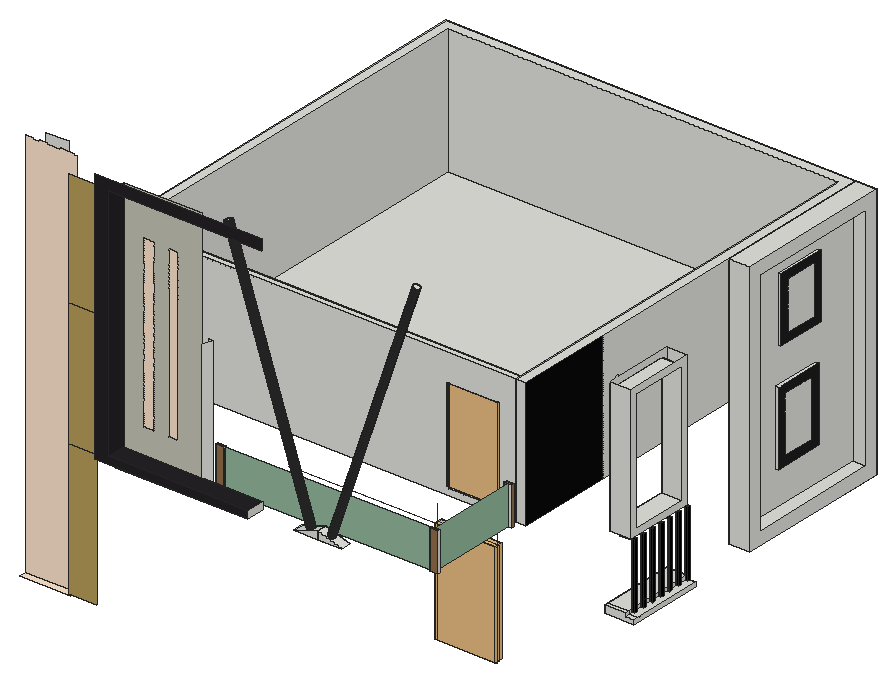
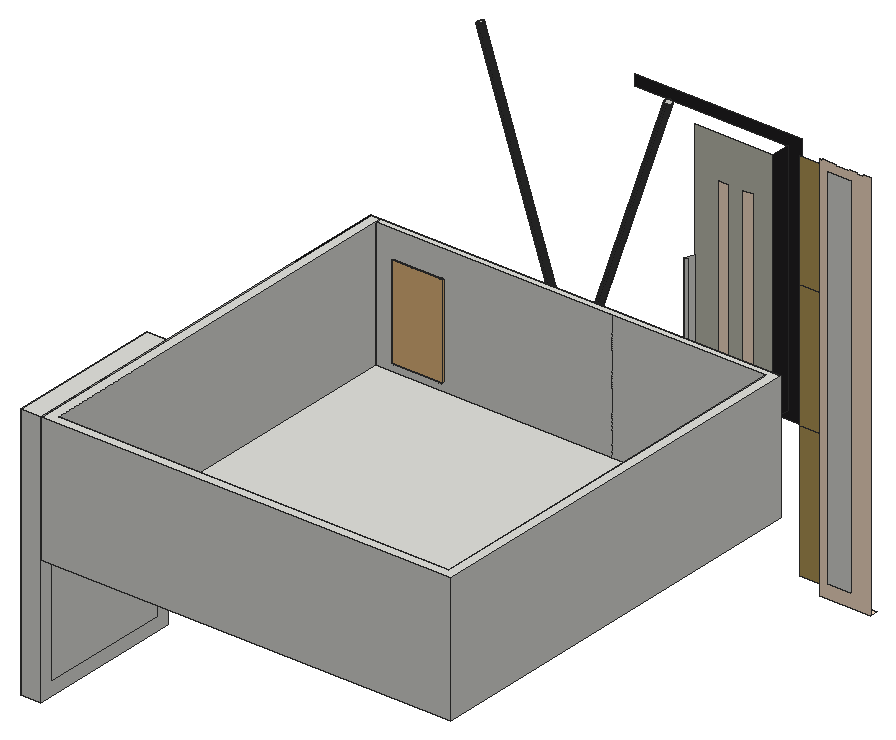
# SketchUp Ruby script. Lengths in inches.
U = 1.inch
M = Sketchup.active_model
def pt(a) = Geom::Point3d.new(a.map { |v| v * U })
def face(e, loops, mat)
  f = e.add_face(loops[0].map { |a| pt(a) })
  loops[1..].each { |l| e.add_face(l.map { |a| pt(a) }).erase! }
  f.material = f.back_material = mat if mat
  f
end
# faces: each face lists its corners as indices into pts; further lists are holes
def faces(e, pts, list, mat = nil) = list.each { |f| face(e, (f[0].is_a?(Array) ? f : [f]).map { |l| l.map { |i| pts[i] } }, mat) }
# xy, xz, yz: faces in a plane at the given z, y or x. An outline is a flat list of corners, or four numbers for a rectangle; further outlines are holes
def ring(l) = l.size == 4 ? [[l[0], l[1]], [l[2], l[1]], [l[2], l[3]], [l[0], l[3]]] : l.each_slice(2).to_a
def flat(e, list, mat, &to3) = list.each { |f| face(e, (f[0].is_a?(Array) ? f : [f]).map { |l| ring(l).map { |u, v| to3.(u, v) } }, mat) }
def xy(e, z, list, mat = nil) = flat(e, list, mat) { |x, y| [x, y, z] }
def xz(e, y, list, mat = nil) = flat(e, list, mat) { |x, z| [x, y, z] }
def yz(e, x, list, mat = nil) = flat(e, list, mat) { |y, z| [x, y, z] }
def lines(e, pts, list) = list.each { |a, b| e.add_line(pt(pts[a]), pt(pts[b])) }
# prism: a flat outline (further loops are holes) pulled along v
def prism(e, loops, v, mat = nil)
  f = face(e, loops, mat); d = Geom::Vector3d.new(v.map { |x| x * U })
  f.pushpull(f.normal.samedirection?(d) ? d.length : -d.length)
end
def box(e, o, s, mat = nil) = prism(e, [[o, [o[0] + s[0], o[1], o[2]], [o[0] + s[0], o[1] + s[1], o[2]], [o[0], o[1] + s[1], o[2]]]], [0, 0, s[2]], mat)
def at(x, y, z, deg = 0) = Geom::Transformation.translation(pt([x, y, z])) * Geom::Transformation.rotation(ORIGIN, Z_AXIS, deg.degrees)
def axes(o, x, y, z) = Geom::Transformation.new([*x, 0, *y, 0, *z, 0, *pt(o).to_a, 1])
def part(name) = M.definitions.add(name)
# library, detail: a bought-in or finely detailed component or shape, given as its bounding box
def library(name, o, s) = part(name).tap { |d| box(d.entities, o, s) }
def detail(e, o, s) = box(e.add_group.entities, o, s)
def put(e, d, t, mat = nil) = e.add_instance(d, t).tap { |i| i.material = mat if mat }
def group(e, t, mat = nil) = e.add_group.tap { |g| g.transformation = t; g.material = mat if mat }.entities
root = M.entities
M.materials.add("C01_Vanilla_Cream").color = [255, 230, 206]
M.materials.add("Glass_Mirror_1").color = [198, 197, 183]
M.materials.add("Glass_Mirror_2").color = [185, 158, 90]
M.materials.add("Glass_Mirror_4").color = [147, 185, 156]
M.materials.add("M08_Obsidian_Black1").color = [30, 30, 30]
M.materials.add("M09_Shadow_Night").color = [0, 0, 0]
M.materials.add("Marble_07_1K").color = [36, 34, 36]
M.materials.add("NERO MARQUINA 02").color = [10, 10, 10]
M.materials.add("Wood_Floor_01_1K").color = [146, 111, 76]
c1 = library("PINTU+6+YA",[0,-0.6875,0],[35.83,8.07,80.71])
xy(root,261.88,[[60,161,107.56,168]],"C01_Vanilla_Cream")
xy(root,269.85,[[444,511.76,463.47,660.3]])
xy(root,275.57,[[444,365.98,471.41,438.64]])
xy(root,279.76,[[463.5,365.98,471.41,370.3],[463.5,370.3,471.41,438.64]])
xy(root,279.99,[[463.57,383.88,466.18,386.33]])
xy(root,281.85,[[444,523.76,450.67,648.3],[450.67,523.76,463.47,648.3]])
xy(root,282.61,[[444,365.98,463.5,370.3],[444,370.3,463.5,438.64]])
xy(root,315.29,[[450.67,557.76,453.74,604.61]])
xy(root,341.81,[[444,372.3125,463.47,438.64]])
xy(root,347.81,[[444,378.3125,463.47,432.64]])
xy(root,384.5,[[450.67,557.76,453.74,604.61]])
xy(root,389.69,[[155.45,154,155.45,168,222,168,222,171,279.03,171,279.03,154],[315.42,162.26,337.89,172.28],[337.89,162.26,360.37,172.28],[230.7,177,238.1,179.5],[431.07,177,438.47,179.5]])
xy(root,389.69,[[431.07,264.56,438.47,267.05]],"Wood_Floor_01_1K")
xy(root,396.93,[[148.69,154,279.03,171]],"Marble_07_1K")
xy(root,418.11,[[450.67,560.84,453.74,607.21]])
xy(root,425.69,[[230.7,177,238.1,179.5],[431.07,177,438.47,179.5]])
xy(root,425.69,[[431.07,264.56,438.47,267.05]],"Wood_Floor_01_1K")
xy(root,461.31,[[444,378.3125,463.47,432.64]])
xy(root,478.5625,[[450.67,560.84,453.74,607.21]])
xy(root,497.69,[[444,523.76,450.67,648.3],[450.67,523.76,463.47,648.3]])
xy(root,509.69,[[444,511.76,463.47,660.3]])
xz(root,154,[[135.55,389.69,279.03,389.69,279.03,396.93,148.69,396.93,148.69,619.42,291.66,619.42,291.66,629.54,135.55,629.54]],"Marble_07_1K")
xz(root,158.24,[[107.56,264.65,133.75,391.05],[107.56,391.05,133.75,509.62],[107.56,509.62,133.75,617.83]],"Glass_Mirror_2")
xz(root,162.26,[[315.42,389.69,337.89,397.24,337.89,389.69],[337.89,389.69,337.89,397.24,360.37,389.69]])
xz(root,168,[[60,261.88,60,629.54,66.39,629.54,66.39,628.54,72.77,628.54,72.77,629.54,79.16,629.54,79.16,628.54,91.93,628.54,91.93,629.54,104.71,629.54,104.71,628.54,107.56,628.54,107.56,261.88]],"C01_Vanilla_Cream")
xz(root,171,[[222,389.69,279.03,396.93]])
xz(root,171,[[191.16,420.48,200.16,579.16],[167.4,420.5,176.8,579.43]],"C01_Vanilla_Cream")
xz(root,171,[[[148.69,396.93,222,619.42],[167.4,420.5,176.8,579.43],[191.16,420.48,200.16,579.16]]],"Glass_Mirror_1")
xz(root,177,[[230.7,389.69,238.1,425.69],[431.07,389.69,438.47,425.69]],"Wood_Floor_01_1K")
xz(root,178.25,[[238.1,389.69,431.07,425.69]],"Glass_Mirror_4")
xz(root,179.5,[[230.7,389.69,238.1,425.69],[431.07,389.69,434.77,425.69],[434.77,389.69,438.47,425.69]])
xz(root,180,[[69,282.89,89.98,629.54]])
xz(root,264.56,[[434.77,389.69,438.47,425.69]])
xz(root,264.56,[[431.07,389.69,434.77,425.69]],"Wood_Floor_01_1K")
xz(root,267.05,[[431.07,389.69,438.47,425.69]],"Wood_Floor_01_1K")
xz(root,365.98,[[444,275.57,471.41,275.57,471.41,279.76,463.5,279.76,463.5,282.61,444,282.61]])
xz(root,372.3125,[[444,341.81,463.47,467.31]])
xz(root,378.3125,[[444,347.81,463.47,461.31]])
xz(root,432.64,[[444,347.81,463.47,461.31]])
xz(root,438.64,[[444,275.57,444,282.61,463.5,282.61,463.5,279.76,471.41,279.76,471.41,275.57],[444,341.81,463.47,467.31]])
xz(root,511.76,[[444,269.85,463.47,509.69]])
xz(root,523.76,[[444,281.85,450.67,497.69],[450.67,281.85,463.47,497.69]])
xz(root,557.76,[[450.67,315.29,453.74,384.5]])
xz(root,560.84,[[450.67,418.11,453.74,478.5625]])
xz(root,604.61,[[450.67,315.29,453.74,384.5]])
xz(root,607.21,[[450.67,418.11,453.74,478.5625]])
xz(root,648.3,[[444,281.85,450.67,497.69],[450.67,281.85,463.47,497.69]])
xz(root,660.3,[[444,269.85,463.47,509.69]])
yz(root,148.69,[[154,396.93,171,619.42]],"Marble_07_1K")
yz(root,230.7,[[177,389.69,179.5,425.69]])
yz(root,238.1,[[177,389.69,178.25,425.69],[178.25,389.69,179.5,425.69]])
yz(root,279.03,[[154,389.69,171,396.93]])
yz(root,337.89,[[162.26,389.69,162.26,397.24,171.26,397.24,172.28,389.69]])
yz(root,431.07,[[177,389.69,178.25,425.69],[178.25,389.69,179.5,425.69]])
yz(root,431.07,[[264.56,389.69,267.05,425.69]],"Wood_Floor_01_1K")
yz(root,434.77,[[179.5,389.69,264.56,425.69]],"Glass_Mirror_4")
yz(root,438.47,[[177,389.69,179.5,425.69]])
yz(root,438.47,[[264.56,389.69,267.05,425.69]],"Wood_Floor_01_1K")
yz(root,444,[[[511.76,269.85,660.3,509.69],[523.76,281.85,648.3,497.69]],[365.98,275.57,438.64,282.61],[523.76,281.85,648.3,497.69],[[372.3125,341.81,372.3125,467.31,378.77,467.31,378.77,468.96,381.22,468.96,381.22,467.31,438.64,467.31,438.64,341.81],[378.3125,347.81,432.64,461.31]]])
yz(root,450.67,[[[523.76,281.85,648.3,497.69],[557.76,315.29,604.61,384.5],[560.84,418.11,607.21,478.5625]]])
yz(root,453.74,[[565.69,323.22,596.68,376.57],[568.23,425.5,599.82,471.17]])
yz(root,453.74,[[[557.76,315.29,604.61,384.5],[565.69,323.22,596.68,376.57]],[[560.84,418.11,607.21,478.5625],[568.23,425.5,599.82,471.17]]],"M08_Obsidian_Black1")
yz(root,463.47,[[[511.76,269.85,660.3,509.69],[523.76,281.85,648.3,497.69]],[[372.3125,341.81,438.64,467.31],[378.3125,347.81,432.64,461.31]]])
yz(root,463.5,[[365.98,279.76,370.3,282.61],[370.3,279.76,438.64,282.61]])
yz(root,471.41,[[365.98,275.57,438.64,279.76]])
p = [[315.42,172.28,389.69],[337.89,171.26,397.24],[337.89,162.26,397.24],[315.42,162.26,389.69],[330.99,168.47,394.92],[330.45,169.08,394.74],
  [329.78,169.53,394.51],[329.01,169.77,394.26],[328.22,169.8,393.99],[327.44,169.62,393.73],[326.74,169.22,393.49],[326.16,168.65,393.3],
  [325.73,167.9375,393.16],[325.5,167.13,393.08],[325.47,166.29,393.07],[325.65,165.47,393.13],[326.02,164.73,393.25],[326.56,164.12,393.4375],
  [327.24,163.67,393.66],[328,163.43,393.92],[328.8,163.4,394.1875],[329.57,163.58,394.45],[330.28,163.98,394.68],[330.86,164.55,394.88],
  [331.28,165.26,395.02],[331.52,166.07,395.1],[331.55,166.91,395.11],[331.37,167.72,395.05],[360.37,172.28,389.69],[360.37,162.26,389.69],
  [225.14,179.94,509.54],[222,171,509.54],[222,171,396.93],[222,171,389.69],[225.14,179.94,389.69],[337.89,172.28,389.69],
  [222,179.95,389.69],[222,179.95,509.54],[350.29,167.52,393.16],[350.43,166.73,393.12],[350.36,165.9375,393.14],[350.1,165.1875,393.23],
  [349.67,164.54,393.375],[349.09,164.02,393.57],[348.4,163.6875,393.8],[347.66,163.55,394.05],[346.91,163.62,394.3],[346.2,163.89,394.54],
  [345.58,164.35,394.75],[345.09,164.96,394.91],[344.77,165.68,395.02],[344.64,166.47,395.06],[344.71,167.26,395.04],[344.97,168.01,394.95],
  [345.4,168.66,394.8],[345.98,169.17,394.61],[346.67,169.51,394.38],[347.41,169.65,394.13],[348.16,169.58,393.88],[348.87,169.31,393.64],
  [349.49,168.85,393.43],[349.98,168.24,393.27],[247.74,165.47,625.1],[248.11,164.73,625.22],[430.04,165.9375,630.38],[429.78,165.1875,630.47],
  [247.5625,166.29,625.04],[430.1,166.73,630.36],[247.59,167.13,625.05],[429.97,167.52,630.4],[247.82,167.9375,625.125],[429.34,164.54,630.61],
  [429.65,168.24,630.51],[248.25,168.65,625.27],[248.66,164.12,625.41],[429.17,168.85,630.67],[248.83,169.22,625.46],[249.33,163.67,625.63],
  [428.76,164.02,630.81],[428.55,169.31,630.88],[249.53,169.62,625.7],[428.08,163.6875,631.04],[427.84,169.58,631.12],[250.09,163.43,625.89],
  [250.31,169.8,625.96],[427.34,163.55,631.29],[250.89,163.4,626.16],[427.09,169.65,631.37],[426.58,163.62,631.54],[251.11,169.77,626.23],
  [426.34,169.51,631.62],[251.67,163.58,626.42],[425.875,163.89,631.78],[251.87,169.53,626.48],[252.37,163.98,626.65],[425.66,169.17,631.85],
  [425.26,164.35,631.98],[252.54,169.08,626.71],[425.08,168.66,632.04],[252.95,164.55,626.85],[424.77,164.96,632.15],[253.09,168.47,626.89],
  [424.65,168.01,632.1875],[253.375,165.26,626.99],[424.45,165.68,632.25],[253.46,167.72,627.02],[253.61,166.07,627.07],[424.32,166.47,632.3],
  [424.39,167.26,632.28],[253.64,166.91,627.08],[213.29,179.94,389.69],[212.95,179.94,389.69],[361.4,273.3,264.64],[361.4,273.3,362.35],
  [417.2,273.3,362.35],[417.2,273.3,264.64],[222,272.89,362.27],[361.4,273.3,377.64],[417.2,273.3,379.69],[361.4,273.3,379.69],
  [361.4,276.53,362.35],[417.2,276.53,362.35],[417.2,276.53,264.64],[361.4,276.53,264.64]]
faces(root,p,[[[0,1,2,3],[4,5,6,7,8,9,10,11,12,13,14,15,16,17,18,19,20,21,22,23,24,25,26,27]],[1,28,29,2],[30,31,32,33,34],[1,0,35],[28,1,35],[34,36,37,30],[38,39,40,41,42,43,44,45,46,47,48,49,50,51,52,53,54,55,56,57,58,59,60,61],[97,101,105,109,106,103,99,94,91,86,83,77,74,63,62,66,68,70,73,76,80,84,89,93],
  [67,69,72,75,79,82,87,90,95,98,102,108,107,104,100,96,92,88,85,81,78,71,65,64]])
faces(root,p,[[16,15,62,63],[41,40,64,65],[15,14,66,62],[40,39,67,64],[14,13,68,66],[39,38,69,67],[13,12,70,68],[42,41,65,71],
  [38,61,72,69],[12,11,73,70],[17,16,63,74],[61,60,75,72],[11,10,76,73],[18,17,74,77],[43,42,71,78],[60,59,79,75],
  [10,9,80,76],[44,43,78,81],[59,58,82,79],[19,18,77,83],[9,8,84,80],[45,44,81,85],[20,19,83,86],[58,57,87,82],
  [46,45,85,88],[8,7,89,84],[57,56,90,87],[21,20,86,91],[47,46,88,92],[7,6,93,89],[22,21,91,94],[56,55,95,90],
  [48,47,92,96],[6,5,97,93],[55,54,98,95],[23,22,94,99],[49,48,96,100],[5,4,101,97],[54,53,102,98],[24,23,99,103],
  [50,49,100,104],[4,27,105,101],[25,24,103,106],[51,50,104,107],[52,51,107,108],[27,26,109,105],[53,52,108,102],[26,25,106,109]],"Marble_07_1K")
lines(root,p,[[110,34],[110,111],[112,113],[113,114],[114,115],[115,112],[113,116],[113,117],[114,118],[117,119],[120,121],[121,122],
  [122,123],[123,120]])
put(root,c1,axes([359.29,273.93,264.64],[1.57176,0,0],[0,0.91463,0],[0,0,1.21055]))
g1 = group(root,at(452.54,436.1875,279.76))
xy(g1,0,[[10.95,0,13.5625,2.45]])
xy(g1,62.05,[[0,0,13.5625,2.45]],"M09_Shadow_Night")
xz(g1,0,[[10.95,0,13.5625,0,13.5625,62.05,0,62.05,0,60.59,10.95,60.59]],"M09_Shadow_Night")
xz(g1,2.45,[[10.95,0,10.95,60.59,0,60.59,0,62.05,13.5625,62.05,13.5625,0]],"M09_Shadow_Night")
yz(g1,10.95,[[0,0,2.45,60.59]])
yz(g1,13.5625,[[0,0,2.45,62.05]],"M09_Shadow_Night")
g2 = group(root,at(452.56,425.73,279.8))
xy(g2,0,[[10.95,0,13.5625,2.45]])
xy(g2,62.05,[[0,0,13.5625,2.45]],"M09_Shadow_Night")
xz(g2,0,[[10.95,0,13.5625,0,13.5625,62.05,0,62.05,0,60.59,10.95,60.59]],"M09_Shadow_Night")
xz(g2,2.45,[[10.95,0,10.95,60.59,0,60.59,0,62.05,13.5625,62.05,13.5625,0]],"M09_Shadow_Night")
yz(g2,10.95,[[0,0,2.45,60.59]])
yz(g2,13.5625,[[0,0,2.45,62.05]],"M09_Shadow_Night")
g3 = group(root,at(452.57,415.27,279.85))
xy(g3,0,[[10.95,0,13.5625,2.45]])
xy(g3,62.05,[[0,0,13.5625,2.45]],"M09_Shadow_Night")
xz(g3,0,[[10.95,0,13.5625,0,13.5625,62.05,0,62.05,0,60.59,10.95,60.59]],"M09_Shadow_Night")
xz(g3,2.45,[[10.95,0,10.95,60.59,0,60.59,0,62.05,13.5625,62.05,13.5625,0]],"M09_Shadow_Night")
yz(g3,10.95,[[0,0,2.45,60.59]])
yz(g3,13.5625,[[0,0,2.45,62.05]],"M09_Shadow_Night")
g4 = group(root,at(452.59,404.81,279.9))
xy(g4,0,[[10.95,0,13.5625,2.45]])
xy(g4,62.05,[[0,0,13.5625,2.45]],"M09_Shadow_Night")
xz(g4,0,[[10.95,0,13.5625,0,13.5625,62.05,0,62.05,0,60.59,10.95,60.59]],"M09_Shadow_Night")
xz(g4,2.45,[[10.95,0,10.95,60.59,0,60.59,0,62.05,13.5625,62.05,13.5625,0]],"M09_Shadow_Night")
yz(g4,10.95,[[0,0,2.45,60.59]])
yz(g4,13.5625,[[0,0,2.45,62.05]],"M09_Shadow_Night")
g5 = group(root,at(452.6,394.35,279.95))
xy(g5,0,[[10.95,0,13.5625,2.45]])
xy(g5,62.05,[[0,0,13.5625,2.45]],"M09_Shadow_Night")
xz(g5,0,[[10.95,0,13.5625,0,13.5625,62.05,0,62.05,0,60.59,10.95,60.59]],"M09_Shadow_Night")
xz(g5,2.45,[[10.95,0,10.95,60.59,0,60.59,0,62.05,13.5625,62.05,13.5625,0]],"M09_Shadow_Night")
yz(g5,10.95,[[0,0,2.45,60.59]])
yz(g5,13.5625,[[0,0,2.45,62.05]],"M09_Shadow_Night")
g6 = group(root,at(452.62,383.88,279.99))
xy(g6,0,[[10.95,0,13.5625,2.45]])
xy(g6,62.05,[[0,0,13.5625,2.45]],"M09_Shadow_Night")
xz(g6,0,[[10.95,0,13.5625,0,13.5625,62.05,0,62.05,0,60.59,10.95,60.59]],"M09_Shadow_Night")
xz(g6,2.45,[[10.95,0,10.95,60.59,0,60.59,0,62.05,13.5625,62.05,13.5625,0]],"M09_Shadow_Night")
yz(g6,10.95,[[0,0,2.45,60.59]])
yz(g6,13.5625,[[0,0,2.45,6.62],[0,6.62,2.45,62.05]],"M09_Shadow_Night")
g7 = group(root,at(452.63,373.42,280.04))
xy(g7,0.07,[[10.95,0,13.5625,2.45]])
xy(g7,62.05,[[0,0,13.5625,2.45]],"M09_Shadow_Night")
xz(g7,0,[[10.95,0.07,13.5625,0.07,13.5625,62.05,0,62.05,0,60.59,10.95,60.59]],"M09_Shadow_Night")
xz(g7,2.45,[[10.95,0.07,10.95,60.59,0,60.59,0,62.05,13.5625,62.05,13.5625,0.07]],"M09_Shadow_Night")
yz(g7,10.95,[[0,0.07,2.45,60.59]])
yz(g7,13.5625,[[0,0.07,2.45,62.05]],"M09_Shadow_Night")
g8 = group(root,at(60,273.3,389.69))
xy(g8,0,[[9,6,375,378]])
xy(g8,5.95,[[312.49,0,358.21,6]])
xy(g8,94.68,[[312.49,0,358.21,6]])
xy(g8,120,[[0,0,375,0,375,6,9,6,9,378,375,378,375,0,384,0,384,387,0,387]])
xz(g8,0,[[9,0,9,120,0,120,0,0.15],[[9,0,375,120],[312.49,5.95,358.21,94.68]],[375,0,384,120]])
xz(g8,6,[[9,0,153,120],[[153,0,375,120],[312.49,5.95,358.21,94.68]]])
xz(g8,378,[[9,0,375,120]])
xz(g8,387,[[0,0,384,120]])
yz(g8,0,[[387,0,0,0.15,0,120,387,120]])
yz(g8,9,[[6,0,378,120]])
yz(g8,312.49,[[0,5.95,6,94.68]])
yz(g8,358.21,[[0,5.95,6,94.68]])
yz(g8,375,[[0,0,6,120],[6,0,378,120]])
yz(g8,384,[[90.12,0,387,120]])
yz(g8,384,[[0,0,90.12,120]],"NERO MARQUINA 02")
put(root,c1,axes([370.91,273.3,397.52],[1.332,0,0],[0,1,0],[0,0,1.07606]))
